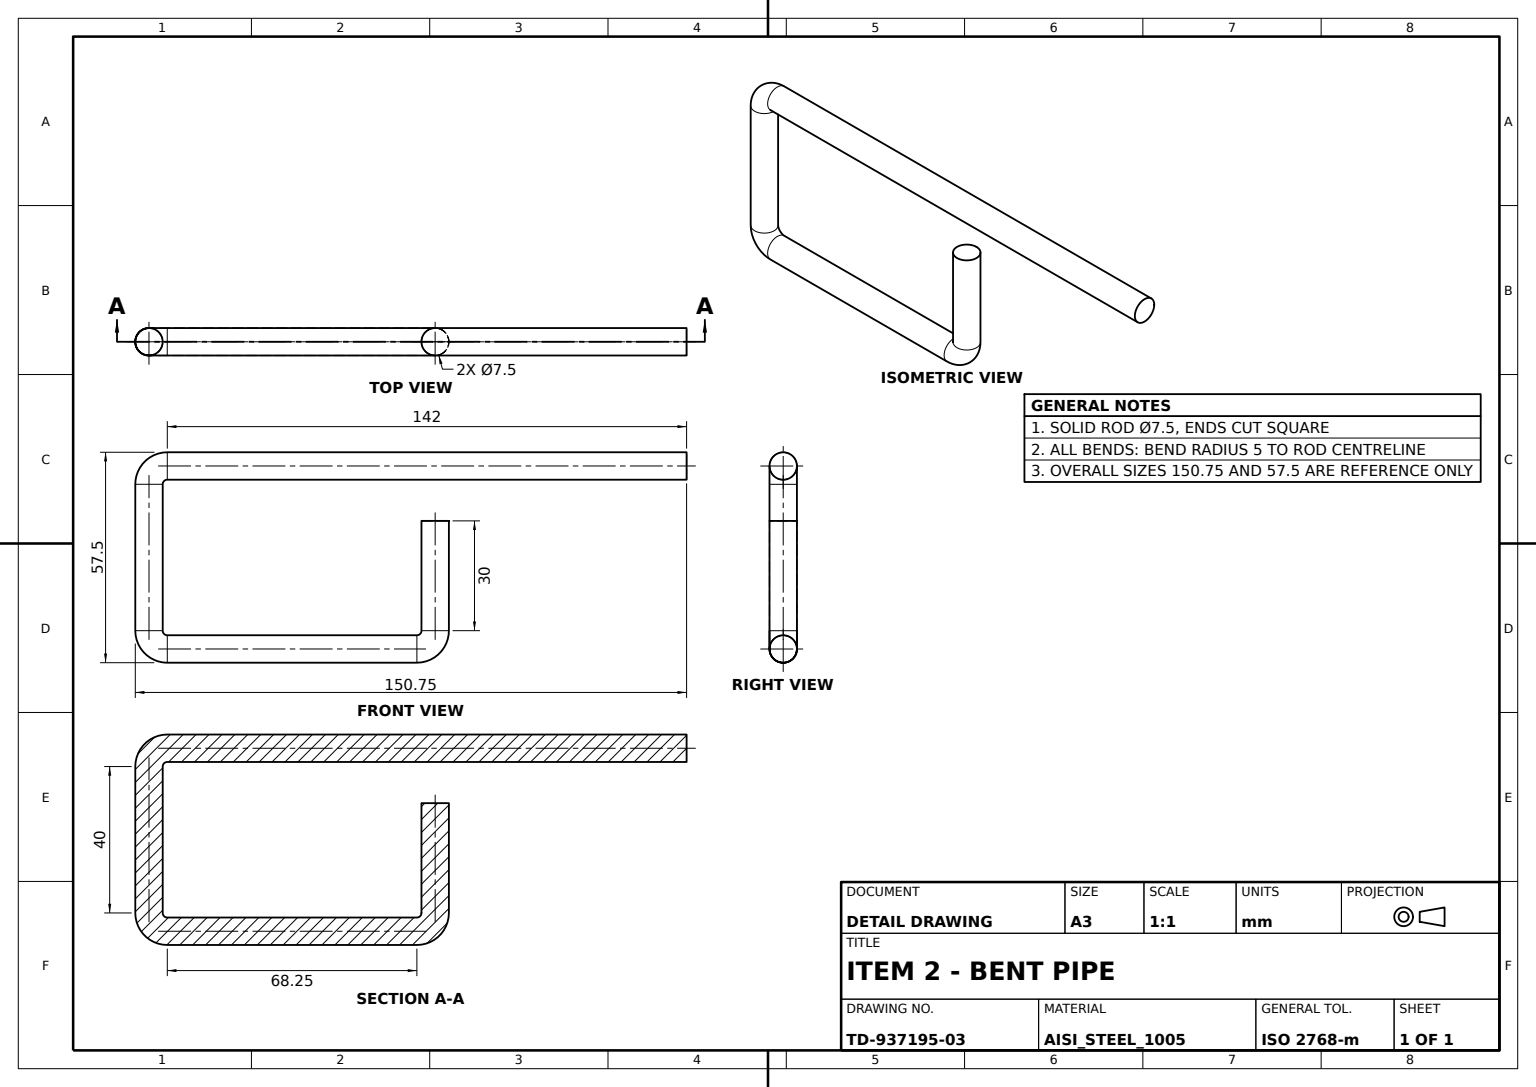
ISO-10303-21;
HEADER;
FILE_DESCRIPTION((''),'2;1');
FILE_NAME('','',(''),(''),'','','');
FILE_SCHEMA(('AUTOMOTIVE_DESIGN'));
ENDSEC;
DATA;
#1=APPLICATION_CONTEXT('');
#2=PRODUCT_CONTEXT('',#1,'mechanical');
#3=PRODUCT('','','',(#2));
#4=PRODUCT_DEFINITION_FORMATION('','',#3);
#5=PRODUCT_DEFINITION_CONTEXT('',#1,'design');
#6=PRODUCT_DEFINITION('','',#4,#5);
#7=PRODUCT_DEFINITION_SHAPE('','',#6);
#8=(LENGTH_UNIT()NAMED_UNIT(*)SI_UNIT(.MILLI.,.METRE.));
#9=(NAMED_UNIT(*)PLANE_ANGLE_UNIT()SI_UNIT($,.RADIAN.));
#10=(NAMED_UNIT(*)SI_UNIT($,.STERADIAN.)SOLID_ANGLE_UNIT());
#11=UNCERTAINTY_MEASURE_WITH_UNIT(LENGTH_MEASURE(0.005),#8,'distance_accuracy_value','');
#12=(GEOMETRIC_REPRESENTATION_CONTEXT(3)GLOBAL_UNCERTAINTY_ASSIGNED_CONTEXT((#11))GLOBAL_UNIT_ASSIGNED_CONTEXT((#8,#9,#10))REPRESENTATION_CONTEXT('',''));
#13=CARTESIAN_POINT('',(-142.,3.75,-50.));
#14=VERTEX_POINT('',#13);
#15=CARTESIAN_POINT('',(-142.,0.,-50.));
#16=DIRECTION('',(-1.,0.,0.));
#17=DIRECTION('',(0.,1.,0.));
#18=AXIS2_PLACEMENT_3D('',#15,#16,#17);
#19=CIRCLE('',#18,3.75);
#20=EDGE_CURVE('',#14,#14,#19,.T.);
#21=ORIENTED_EDGE('',*,*,#20,.T.);
#22=EDGE_LOOP('',(#21));
#23=FACE_BOUND('',#22,.T.);
#24=CARTESIAN_POINT('',(-147.,3.75,-45.));
#25=VERTEX_POINT('',#24);
#26=CARTESIAN_POINT('',(-147.,0.,-45.));
#27=DIRECTION('',(0.,0.,1.));
#28=AXIS2_PLACEMENT_3D('',#26,#27,#17);
#29=CIRCLE('',#28,3.75);
#30=EDGE_CURVE('',#25,#25,#29,.T.);
#31=ORIENTED_EDGE('',*,*,#30,.F.);
#32=EDGE_LOOP('',(#31));
#33=FACE_BOUND('',#32,.T.);
#34=CARTESIAN_POINT('',(-142.,0.,-45.));
#35=DIRECTION('',(0.,-1.,0.));
#36=DIRECTION('',(0.,0.,-1.));
#37=AXIS2_PLACEMENT_3D('',#34,#35,#36);
#38=TOROIDAL_SURFACE('',#37,5.,3.75);
#39=ADVANCED_FACE('',(#23,#33),#38,.T.);
#40=CARTESIAN_POINT('',(0.,3.75,0.));
#41=VERTEX_POINT('',#40);
#42=CARTESIAN_POINT('',(0.,0.,0.));
#43=DIRECTION('',(1.,0.,0.));
#44=AXIS2_PLACEMENT_3D('',#42,#43,#17);
#45=CIRCLE('',#44,3.75);
#46=EDGE_CURVE('',#41,#41,#45,.T.);
#47=ORIENTED_EDGE('',*,*,#46,.T.);
#48=EDGE_LOOP('',(#47));
#49=FACE_BOUND('',#48,.T.);
#50=AXIS2_PLACEMENT_3D('',#42,#43,#36);
#51=PLANE('',#50);
#52=ADVANCED_FACE('',(#49),#51,.T.);
#53=CARTESIAN_POINT('',(-142.,3.75,0.));
#54=VERTEX_POINT('',#53);
#55=CARTESIAN_POINT('',(-142.,0.,0.));
#56=AXIS2_PLACEMENT_3D('',#55,#43,#17);
#57=CIRCLE('',#56,3.75);
#58=EDGE_CURVE('',#54,#54,#57,.T.);
#59=ORIENTED_EDGE('',*,*,#58,.F.);
#60=EDGE_LOOP('',(#59));
#61=FACE_BOUND('',#60,.T.);
#62=CARTESIAN_POINT('',(-147.,3.75,-5.));
#63=VERTEX_POINT('',#62);
#64=CARTESIAN_POINT('',(-147.,0.,-5.));
#65=AXIS2_PLACEMENT_3D('',#64,#27,#17);
#66=CIRCLE('',#65,3.75);
#67=EDGE_CURVE('',#63,#63,#66,.T.);
#68=ORIENTED_EDGE('',*,*,#67,.T.);
#69=EDGE_LOOP('',(#68));
#70=FACE_BOUND('',#69,.T.);
#71=CARTESIAN_POINT('',(-142.,0.,-5.));
#72=AXIS2_PLACEMENT_3D('',#71,#35,#36);
#73=TOROIDAL_SURFACE('',#72,5.,3.75);
#74=ADVANCED_FACE('',(#61,#70),#73,.T.);
#75=ORIENTED_EDGE('',*,*,#20,.F.);
#76=EDGE_LOOP('',(#75));
#77=FACE_BOUND('',#76,.T.);
#78=CARTESIAN_POINT('',(-73.75,3.75,-50.));
#79=VERTEX_POINT('',#78);
#80=CARTESIAN_POINT('',(-73.75,0.,-50.));
#81=AXIS2_PLACEMENT_3D('',#80,#16,#17);
#82=CIRCLE('',#81,3.75);
#83=EDGE_CURVE('',#79,#79,#82,.T.);
#84=ORIENTED_EDGE('',*,*,#83,.T.);
#85=EDGE_LOOP('',(#84));
#86=FACE_BOUND('',#85,.T.);
#87=AXIS2_PLACEMENT_3D('',#15,#43,#36);
#88=CYLINDRICAL_SURFACE('',#87,3.75);
#89=ADVANCED_FACE('',(#77,#86),#88,.T.);
#90=CARTESIAN_POINT('',(-68.75,3.75,-15.));
#91=VERTEX_POINT('',#90);
#92=CARTESIAN_POINT('',(-68.75,0.,-15.));
#93=AXIS2_PLACEMENT_3D('',#92,#36,#17);
#94=CIRCLE('',#93,3.75);
#95=EDGE_CURVE('',#91,#91,#94,.T.);
#96=ORIENTED_EDGE('',*,*,#95,.F.);
#97=EDGE_LOOP('',(#96));
#98=FACE_BOUND('',#97,.T.);
#99=AXIS2_PLACEMENT_3D('',#92,#36,#16);
#100=PLANE('',#99);
#101=ADVANCED_FACE('',(#98),#100,.F.);
#102=CARTESIAN_POINT('',(-68.75,3.75,-45.));
#103=VERTEX_POINT('',#102);
#104=CARTESIAN_POINT('',(-68.75,0.,-45.));
#105=AXIS2_PLACEMENT_3D('',#104,#36,#17);
#106=CIRCLE('',#105,3.75);
#107=EDGE_CURVE('',#103,#103,#106,.T.);
#108=ORIENTED_EDGE('',*,*,#107,.F.);
#109=EDGE_LOOP('',(#108));
#110=FACE_BOUND('',#109,.T.);
#111=ORIENTED_EDGE('',*,*,#95,.T.);
#112=EDGE_LOOP('',(#111));
#113=FACE_BOUND('',#112,.T.);
#114=AXIS2_PLACEMENT_3D('',#104,#27,#43);
#115=CYLINDRICAL_SURFACE('',#114,3.75);
#116=ADVANCED_FACE('',(#110,#113),#115,.T.);
#117=ORIENTED_EDGE('',*,*,#83,.F.);
#118=EDGE_LOOP('',(#117));
#119=FACE_BOUND('',#118,.T.);
#120=ORIENTED_EDGE('',*,*,#107,.T.);
#121=EDGE_LOOP('',(#120));
#122=FACE_BOUND('',#121,.T.);
#123=CARTESIAN_POINT('',(-73.75,0.,-45.));
#124=AXIS2_PLACEMENT_3D('',#123,#35,#36);
#125=TOROIDAL_SURFACE('',#124,5.,3.75);
#126=ADVANCED_FACE('',(#119,#122),#125,.T.);
#127=ORIENTED_EDGE('',*,*,#30,.T.);
#128=EDGE_LOOP('',(#127));
#129=FACE_BOUND('',#128,.T.);
#130=ORIENTED_EDGE('',*,*,#67,.F.);
#131=EDGE_LOOP('',(#130));
#132=FACE_BOUND('',#131,.T.);
#133=AXIS2_PLACEMENT_3D('',#64,#36,#16);
#134=CYLINDRICAL_SURFACE('',#133,3.75);
#135=ADVANCED_FACE('',(#129,#132),#134,.T.);
#136=ORIENTED_EDGE('',*,*,#58,.T.);
#137=EDGE_LOOP('',(#136));
#138=FACE_BOUND('',#137,.T.);
#139=ORIENTED_EDGE('',*,*,#46,.F.);
#140=EDGE_LOOP('',(#139));
#141=FACE_BOUND('',#140,.T.);
#142=AXIS2_PLACEMENT_3D('',#55,#43,#36);
#143=CYLINDRICAL_SURFACE('',#142,3.75);
#144=ADVANCED_FACE('',(#138,#141),#143,.T.);
#145=CLOSED_SHELL('',(#39,#52,#74,#89,#101,#116,#126,#135,#144));
#146=MANIFOLD_SOLID_BREP('',#145);
#147=ADVANCED_BREP_SHAPE_REPRESENTATION('',(#146),#12);
#148=SHAPE_DEFINITION_REPRESENTATION(#7,#147);
ENDSEC;
END-ISO-10303-21;
